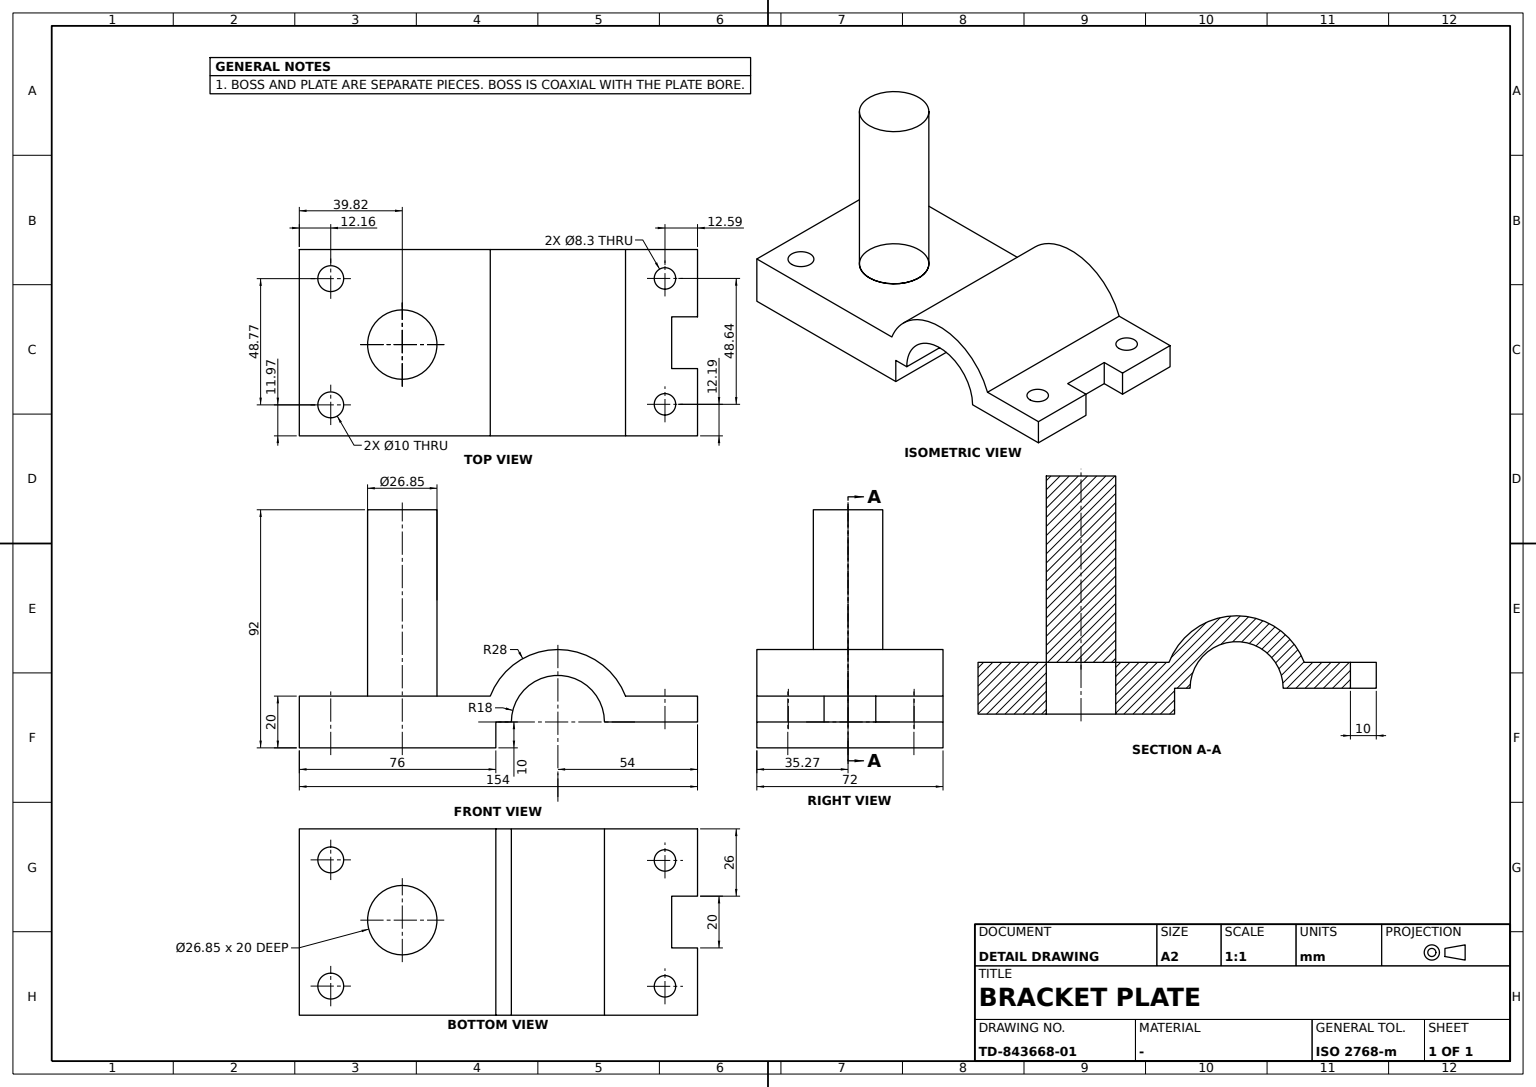
ISO-10303-21;
HEADER;
FILE_DESCRIPTION((''),'2;1');
FILE_NAME('','',(''),(''),'','','');
FILE_SCHEMA(('AUTOMOTIVE_DESIGN'));
ENDSEC;
DATA;
#1=APPLICATION_CONTEXT('');
#2=PRODUCT_CONTEXT('',#1,'mechanical');
#3=PRODUCT('','','',(#2));
#4=PRODUCT_DEFINITION_FORMATION('','',#3);
#5=PRODUCT_DEFINITION_CONTEXT('',#1,'design');
#6=PRODUCT_DEFINITION('','',#4,#5);
#7=PRODUCT_DEFINITION_SHAPE('','',#6);
#8=(LENGTH_UNIT()NAMED_UNIT(*)SI_UNIT(.MILLI.,.METRE.));
#9=(NAMED_UNIT(*)PLANE_ANGLE_UNIT()SI_UNIT($,.RADIAN.));
#10=(NAMED_UNIT(*)SI_UNIT($,.STERADIAN.)SOLID_ANGLE_UNIT());
#11=UNCERTAINTY_MEASURE_WITH_UNIT(LENGTH_MEASURE(0.005),#8,'distance_accuracy_value','');
#12=(GEOMETRIC_REPRESENTATION_CONTEXT(3)GLOBAL_UNCERTAINTY_ASSIGNED_CONTEXT((#11))GLOBAL_UNIT_ASSIGNED_CONTEXT((#8,#9,#10))REPRESENTATION_CONTEXT('',''));
#13=CARTESIAN_POINT('',(-21.846565,-37.180111,82.));
#14=VERTEX_POINT('',#13);
#15=CARTESIAN_POINT('',(-35.26936,-37.180111,82.));
#16=DIRECTION('',(0.,0.,1.));
#17=DIRECTION('',(1.,0.,0.));
#18=AXIS2_PLACEMENT_3D('',#15,#16,#17);
#19=CIRCLE('',#18,13.422795);
#20=EDGE_CURVE('',#14,#14,#19,.T.);
#21=ORIENTED_EDGE('',*,*,#20,.T.);
#22=EDGE_LOOP('',(#21));
#23=FACE_BOUND('',#22,.T.);
#24=CARTESIAN_POINT('',(0.,0.,82.));
#25=AXIS2_PLACEMENT_3D('',#24,#16,#17);
#26=PLANE('',#25);
#27=ADVANCED_FACE('',(#23),#26,.T.);
#28=CARTESIAN_POINT('',(-21.846565,-37.180111,10.));
#29=VERTEX_POINT('',#28);
#30=CARTESIAN_POINT('',(-35.26936,-37.180111,10.));
#31=AXIS2_PLACEMENT_3D('',#30,#16,#17);
#32=CIRCLE('',#31,13.422795);
#33=EDGE_CURVE('',#29,#29,#32,.T.);
#34=ORIENTED_EDGE('',*,*,#33,.F.);
#35=EDGE_LOOP('',(#34));
#36=FACE_BOUND('',#35,.T.);
#37=CARTESIAN_POINT('',(0.,49.153394,10.));
#38=DIRECTION('',(0.,1.,0.));
#39=AXIS2_PLACEMENT_3D('',#37,#16,#38);
#40=PLANE('',#39);
#41=ADVANCED_FACE('',(#36),#40,.F.);
#42=ORIENTED_EDGE('',*,*,#33,.T.);
#43=EDGE_LOOP('',(#42));
#44=FACE_BOUND('',#43,.T.);
#45=ORIENTED_EDGE('',*,*,#20,.F.);
#46=EDGE_LOOP('',(#45));
#47=FACE_BOUND('',#46,.T.);
#48=CARTESIAN_POINT('',(-35.26936,-37.180111,46.));
#49=AXIS2_PLACEMENT_3D('',#48,#16,#17);
#50=CYLINDRICAL_SURFACE('',#49,13.422795);
#51=ADVANCED_FACE('',(#44,#47),#50,.T.);
#52=CLOSED_SHELL('',(#27,#41,#51));
#53=MANIFOLD_SOLID_BREP('',#52);
#54=CARTESIAN_POINT('',(-48.692154,-37.180111,-10.));
#55=VERTEX_POINT('',#54);
#56=CARTESIAN_POINT('',(-35.26936,-37.180111,-10.));
#57=DIRECTION('',(0.,0.,-1.));
#58=DIRECTION('',(-1.,0.,0.));
#59=AXIS2_PLACEMENT_3D('',#56,#57,#58);
#60=CIRCLE('',#59,13.422795);
#61=EDGE_CURVE('',#55,#55,#60,.T.);
#62=ORIENTED_EDGE('',*,*,#61,.T.);
#63=EDGE_LOOP('',(#62));
#64=FACE_BOUND('',#63,.T.);
#65=VERTEX_POINT('',#28);
#66=EDGE_CURVE('',#65,#65,#32,.T.);
#67=ORIENTED_EDGE('',*,*,#66,.T.);
#68=EDGE_LOOP('',(#67));
#69=FACE_BOUND('',#68,.T.);
#70=ADVANCED_FACE('',(#64,#69),#50,.F.);
#71=CARTESIAN_POINT('',(0.,-1.,-10.));
#72=VERTEX_POINT('',#71);
#73=CARTESIAN_POINT('',(-72.,-1.,-10.));
#74=VERTEX_POINT('',#73);
#75=VECTOR('',#58,1000.);
#76=LINE('',#71,#75);
#77=EDGE_CURVE('',#72,#74,#76,.T.);
#78=ORIENTED_EDGE('',*,*,#77,.T.);
#79=CARTESIAN_POINT('',(-72.,-1.,0.));
#80=VERTEX_POINT('',#79);
#81=VECTOR('',#57,1000.);
#82=LINE('',#79,#81);
#83=EDGE_CURVE('',#80,#74,#82,.T.);
#84=ORIENTED_EDGE('',*,*,#83,.F.);
#85=CARTESIAN_POINT('',(0.,-1.,0.));
#86=VERTEX_POINT('',#85);
#87=LINE('',#85,#75);
#88=EDGE_CURVE('',#86,#80,#87,.T.);
#89=ORIENTED_EDGE('',*,*,#88,.F.);
#90=LINE('',#85,#81);
#91=EDGE_CURVE('',#86,#72,#90,.T.);
#92=ORIENTED_EDGE('',*,*,#91,.T.);
#93=EDGE_LOOP('',(#78,#84,#89,#92));
#94=FACE_BOUND('',#93,.T.);
#95=AXIS2_PLACEMENT_3D('',#85,#38,#57);
#96=PLANE('',#95);
#97=ADVANCED_FACE('',(#94),#96,.T.);
#98=CARTESIAN_POINT('',(0.,-77.,-10.));
#99=VERTEX_POINT('',#98);
#100=CARTESIAN_POINT('',(0.,-77.,10.));
#101=VERTEX_POINT('',#100);
#102=VECTOR('',#16,1000.);
#103=LINE('',#98,#102);
#104=EDGE_CURVE('',#99,#101,#103,.T.);
#105=ORIENTED_EDGE('',*,*,#104,.F.);
#106=DIRECTION('',(0.,-1.,0.));
#107=VECTOR('',#106,1000.);
#108=LINE('',#71,#107);
#109=EDGE_CURVE('',#72,#99,#108,.T.);
#110=ORIENTED_EDGE('',*,*,#109,.F.);
#111=ORIENTED_EDGE('',*,*,#91,.F.);
#112=CARTESIAN_POINT('',(0.,5.,0.));
#113=VERTEX_POINT('',#112);
#114=LINE('',#112,#107);
#115=EDGE_CURVE('',#113,#86,#114,.T.);
#116=ORIENTED_EDGE('',*,*,#115,.F.);
#117=CARTESIAN_POINT('',(0.,41.,0.));
#118=VERTEX_POINT('',#117);
#119=CARTESIAN_POINT('',(0.,23.,0.));
#120=AXIS2_PLACEMENT_3D('',#119,#17,#57);
#121=CIRCLE('',#120,18.);
#122=EDGE_CURVE('',#118,#113,#121,.T.);
#123=ORIENTED_EDGE('',*,*,#122,.F.);
#124=CARTESIAN_POINT('',(0.,77.,0.));
#125=VERTEX_POINT('',#124);
#126=EDGE_CURVE('',#125,#118,#114,.T.);
#127=ORIENTED_EDGE('',*,*,#126,.F.);
#128=CARTESIAN_POINT('',(0.,77.,10.));
#129=VERTEX_POINT('',#128);
#130=LINE('',#128,#81);
#131=EDGE_CURVE('',#129,#125,#130,.T.);
#132=ORIENTED_EDGE('',*,*,#131,.F.);
#133=VERTEX_POINT('',#37);
#134=VECTOR('',#38,1000.);
#135=LINE('',#37,#134);
#136=EDGE_CURVE('',#133,#129,#135,.T.);
#137=ORIENTED_EDGE('',*,*,#136,.F.);
#138=CARTESIAN_POINT('',(0.,-3.153394,10.));
#139=VERTEX_POINT('',#138);
#140=CIRCLE('',#120,28.);
#141=EDGE_CURVE('',#133,#139,#140,.T.);
#142=ORIENTED_EDGE('',*,*,#141,.T.);
#143=EDGE_CURVE('',#101,#139,#135,.T.);
#144=ORIENTED_EDGE('',*,*,#143,.F.);
#145=EDGE_LOOP('',(#105,#110,#111,#116,#123,#127,#132,#137,#142,#144));
#146=FACE_BOUND('',#145,.T.);
#147=CARTESIAN_POINT('',(0.,0.,0.));
#148=AXIS2_PLACEMENT_3D('',#147,#17,#38);
#149=PLANE('',#148);
#150=ADVANCED_FACE('',(#146),#149,.T.);
#151=CARTESIAN_POINT('',(-64.984131,64.410873,0.));
#152=VERTEX_POINT('',#151);
#153=CARTESIAN_POINT('',(-60.834221,64.410873,0.));
#154=AXIS2_PLACEMENT_3D('',#153,#57,#58);
#155=CIRCLE('',#154,4.14991);
#156=EDGE_CURVE('',#152,#152,#155,.T.);
#157=ORIENTED_EDGE('',*,*,#156,.T.);
#158=EDGE_LOOP('',(#157));
#159=FACE_BOUND('',#158,.T.);
#160=CARTESIAN_POINT('',(-56.684311,64.410873,10.));
#161=VERTEX_POINT('',#160);
#162=CARTESIAN_POINT('',(-60.834221,64.410873,10.));
#163=AXIS2_PLACEMENT_3D('',#162,#16,#17);
#164=CIRCLE('',#163,4.14991);
#165=EDGE_CURVE('',#161,#161,#164,.T.);
#166=ORIENTED_EDGE('',*,*,#165,.T.);
#167=EDGE_LOOP('',(#166));
#168=FACE_BOUND('',#167,.T.);
#169=CARTESIAN_POINT('',(-60.834221,64.410873,-26.));
#170=AXIS2_PLACEMENT_3D('',#169,#16,#17);
#171=CYLINDRICAL_SURFACE('',#170,4.14991);
#172=ADVANCED_FACE('',(#159,#168),#171,.F.);
#173=ORIENTED_EDGE('',*,*,#109,.T.);
#174=CARTESIAN_POINT('',(-72.,-77.,-10.));
#175=VERTEX_POINT('',#174);
#176=LINE('',#98,#75);
#177=EDGE_CURVE('',#99,#175,#176,.T.);
#178=ORIENTED_EDGE('',*,*,#177,.T.);
#179=LINE('',#73,#107);
#180=EDGE_CURVE('',#74,#175,#179,.T.);
#181=ORIENTED_EDGE('',*,*,#180,.F.);
#182=ORIENTED_EDGE('',*,*,#77,.F.);
#183=EDGE_LOOP('',(#173,#178,#181,#182));
#184=FACE_BOUND('',#183,.T.);
#185=ORIENTED_EDGE('',*,*,#61,.F.);
#186=EDGE_LOOP('',(#185));
#187=FACE_BOUND('',#186,.T.);
#188=CARTESIAN_POINT('',(-16.97486,-64.842331,-10.));
#189=VERTEX_POINT('',#188);
#190=CARTESIAN_POINT('',(-11.97486,-64.842331,-10.));
#191=AXIS2_PLACEMENT_3D('',#190,#57,#58);
#192=CIRCLE('',#191,5.);
#193=EDGE_CURVE('',#189,#189,#192,.T.);
#194=ORIENTED_EDGE('',*,*,#193,.F.);
#195=EDGE_LOOP('',(#194));
#196=FACE_BOUND('',#195,.T.);
#197=CARTESIAN_POINT('',(-65.747715,-64.842331,-10.));
#198=VERTEX_POINT('',#197);
#199=CARTESIAN_POINT('',(-60.747715,-64.842331,-10.));
#200=AXIS2_PLACEMENT_3D('',#199,#57,#58);
#201=CIRCLE('',#200,5.);
#202=EDGE_CURVE('',#198,#198,#201,.T.);
#203=ORIENTED_EDGE('',*,*,#202,.F.);
#204=EDGE_LOOP('',(#203));
#205=FACE_BOUND('',#204,.T.);
#206=AXIS2_PLACEMENT_3D('',#71,#57,#106);
#207=PLANE('',#206);
#208=ADVANCED_FACE('',(#184,#187,#196,#205),#207,.T.);
#209=ORIENTED_EDGE('',*,*,#122,.T.);
#210=CARTESIAN_POINT('',(-72.,5.,0.));
#211=VERTEX_POINT('',#210);
#212=VECTOR('',#17,1000.);
#213=LINE('',#112,#212);
#214=EDGE_CURVE('',#113,#211,#213,.F.);
#215=ORIENTED_EDGE('',*,*,#214,.T.);
#216=CARTESIAN_POINT('',(-72.,41.,0.));
#217=VERTEX_POINT('',#216);
#218=CARTESIAN_POINT('',(-72.,23.,0.));
#219=AXIS2_PLACEMENT_3D('',#218,#17,#57);
#220=CIRCLE('',#219,18.);
#221=EDGE_CURVE('',#217,#211,#220,.T.);
#222=ORIENTED_EDGE('',*,*,#221,.F.);
#223=LINE('',#117,#212);
#224=EDGE_CURVE('',#118,#217,#223,.F.);
#225=ORIENTED_EDGE('',*,*,#224,.F.);
#226=EDGE_LOOP('',(#209,#215,#222,#225));
#227=FACE_BOUND('',#226,.T.);
#228=CARTESIAN_POINT('',(-36.,23.,0.));
#229=AXIS2_PLACEMENT_3D('',#228,#17,#38);
#230=CYLINDRICAL_SURFACE('',#229,18.);
#231=ADVANCED_FACE('',(#227),#230,.F.);
#232=CARTESIAN_POINT('',(-55.747715,-64.842331,10.));
#233=VERTEX_POINT('',#232);
#234=CARTESIAN_POINT('',(-60.747715,-64.842331,10.));
#235=AXIS2_PLACEMENT_3D('',#234,#16,#17);
#236=CIRCLE('',#235,5.);
#237=EDGE_CURVE('',#233,#233,#236,.T.);
#238=ORIENTED_EDGE('',*,*,#237,.T.);
#239=EDGE_LOOP('',(#238));
#240=FACE_BOUND('',#239,.T.);
#241=ORIENTED_EDGE('',*,*,#202,.T.);
#242=EDGE_LOOP('',(#241));
#243=FACE_BOUND('',#242,.T.);
#244=CARTESIAN_POINT('',(-60.747715,-64.842331,-26.));
#245=AXIS2_PLACEMENT_3D('',#244,#16,#17);
#246=CYLINDRICAL_SURFACE('',#245,5.);
#247=ADVANCED_FACE('',(#240,#243),#246,.F.);
#248=CARTESIAN_POINT('',(-72.,-77.,10.));
#249=VERTEX_POINT('',#248);
#250=LINE('',#174,#102);
#251=EDGE_CURVE('',#175,#249,#250,.T.);
#252=ORIENTED_EDGE('',*,*,#251,.F.);
#253=ORIENTED_EDGE('',*,*,#177,.F.);
#254=ORIENTED_EDGE('',*,*,#104,.T.);
#255=LINE('',#100,#75);
#256=EDGE_CURVE('',#101,#249,#255,.T.);
#257=ORIENTED_EDGE('',*,*,#256,.T.);
#258=EDGE_LOOP('',(#252,#253,#254,#257));
#259=FACE_BOUND('',#258,.T.);
#260=AXIS2_PLACEMENT_3D('',#98,#106,#16);
#261=PLANE('',#260);
#262=ADVANCED_FACE('',(#259),#261,.T.);
#263=ORIENTED_EDGE('',*,*,#193,.T.);
#264=EDGE_LOOP('',(#263));
#265=FACE_BOUND('',#264,.T.);
#266=CARTESIAN_POINT('',(-6.97486,-64.842331,10.));
#267=VERTEX_POINT('',#266);
#268=CARTESIAN_POINT('',(-11.97486,-64.842331,10.));
#269=AXIS2_PLACEMENT_3D('',#268,#16,#17);
#270=CIRCLE('',#269,5.);
#271=EDGE_CURVE('',#267,#267,#270,.T.);
#272=ORIENTED_EDGE('',*,*,#271,.T.);
#273=EDGE_LOOP('',(#272));
#274=FACE_BOUND('',#273,.T.);
#275=CARTESIAN_POINT('',(-11.97486,-64.842331,-26.));
#276=AXIS2_PLACEMENT_3D('',#275,#16,#17);
#277=CYLINDRICAL_SURFACE('',#276,5.);
#278=ADVANCED_FACE('',(#265,#274),#277,.F.);
#279=ORIENTED_EDGE('',*,*,#271,.F.);
#280=EDGE_LOOP('',(#279));
#281=FACE_BOUND('',#280,.T.);
#282=ORIENTED_EDGE('',*,*,#256,.F.);
#283=ORIENTED_EDGE('',*,*,#143,.T.);
#284=CARTESIAN_POINT('',(-72.,-3.153394,10.));
#285=VERTEX_POINT('',#284);
#286=LINE('',#138,#212);
#287=EDGE_CURVE('',#139,#285,#286,.F.);
#288=ORIENTED_EDGE('',*,*,#287,.T.);
#289=CARTESIAN_POINT('',(-72.,49.153394,10.));
#290=LINE('',#289,#134);
#291=EDGE_CURVE('',#249,#285,#290,.T.);
#292=ORIENTED_EDGE('',*,*,#291,.F.);
#293=EDGE_LOOP('',(#282,#283,#288,#292));
#294=FACE_BOUND('',#293,.T.);
#295=ORIENTED_EDGE('',*,*,#66,.F.);
#296=EDGE_LOOP('',(#295));
#297=FACE_BOUND('',#296,.T.);
#298=ORIENTED_EDGE('',*,*,#237,.F.);
#299=EDGE_LOOP('',(#298));
#300=FACE_BOUND('',#299,.T.);
#301=ADVANCED_FACE('',(#281,#294,#297,#300),#40,.T.);
#302=ORIENTED_EDGE('',*,*,#287,.F.);
#303=ORIENTED_EDGE('',*,*,#141,.F.);
#304=VERTEX_POINT('',#289);
#305=LINE('',#37,#212);
#306=EDGE_CURVE('',#133,#304,#305,.F.);
#307=ORIENTED_EDGE('',*,*,#306,.T.);
#308=CIRCLE('',#219,28.);
#309=EDGE_CURVE('',#304,#285,#308,.T.);
#310=ORIENTED_EDGE('',*,*,#309,.T.);
#311=EDGE_LOOP('',(#302,#303,#307,#310));
#312=FACE_BOUND('',#311,.T.);
#313=CYLINDRICAL_SURFACE('',#229,28.);
#314=ADVANCED_FACE('',(#312),#313,.T.);
#315=CARTESIAN_POINT('',(-26.,77.,0.));
#316=VERTEX_POINT('',#315);
#317=LINE('',#124,#75);
#318=EDGE_CURVE('',#125,#316,#317,.T.);
#319=ORIENTED_EDGE('',*,*,#318,.T.);
#320=CARTESIAN_POINT('',(-26.,77.,10.));
#321=VERTEX_POINT('',#320);
#322=LINE('',#320,#81);
#323=EDGE_CURVE('',#321,#316,#322,.T.);
#324=ORIENTED_EDGE('',*,*,#323,.F.);
#325=LINE('',#128,#75);
#326=EDGE_CURVE('',#129,#321,#325,.T.);
#327=ORIENTED_EDGE('',*,*,#326,.F.);
#328=ORIENTED_EDGE('',*,*,#131,.T.);
#329=EDGE_LOOP('',(#319,#324,#327,#328));
#330=FACE_BOUND('',#329,.T.);
#331=AXIS2_PLACEMENT_3D('',#128,#38,#57);
#332=PLANE('',#331);
#333=ADVANCED_FACE('',(#330),#332,.T.);
#334=CARTESIAN_POINT('',(-26.,67.,10.));
#335=VERTEX_POINT('',#334);
#336=CARTESIAN_POINT('',(-26.,67.,0.));
#337=VERTEX_POINT('',#336);
#338=LINE('',#334,#81);
#339=EDGE_CURVE('',#335,#337,#338,.T.);
#340=ORIENTED_EDGE('',*,*,#339,.T.);
#341=CARTESIAN_POINT('',(-46.,67.,0.));
#342=VERTEX_POINT('',#341);
#343=CARTESIAN_POINT('',(0.,67.,0.));
#344=LINE('',#343,#75);
#345=EDGE_CURVE('',#337,#342,#344,.T.);
#346=ORIENTED_EDGE('',*,*,#345,.T.);
#347=CARTESIAN_POINT('',(-46.,67.,10.));
#348=VERTEX_POINT('',#347);
#349=LINE('',#347,#81);
#350=EDGE_CURVE('',#348,#342,#349,.T.);
#351=ORIENTED_EDGE('',*,*,#350,.F.);
#352=LINE('',#334,#75);
#353=EDGE_CURVE('',#335,#348,#352,.T.);
#354=ORIENTED_EDGE('',*,*,#353,.F.);
#355=EDGE_LOOP('',(#340,#346,#351,#354));
#356=FACE_BOUND('',#355,.T.);
#357=AXIS2_PLACEMENT_3D('',#334,#106,#58);
#358=PLANE('',#357);
#359=ADVANCED_FACE('',(#356),#358,.F.);
#360=ORIENTED_EDGE('',*,*,#339,.F.);
#361=LINE('',#320,#107);
#362=EDGE_CURVE('',#321,#335,#361,.T.);
#363=ORIENTED_EDGE('',*,*,#362,.F.);
#364=ORIENTED_EDGE('',*,*,#323,.T.);
#365=CARTESIAN_POINT('',(-26.,5.,0.));
#366=LINE('',#365,#107);
#367=EDGE_CURVE('',#316,#337,#366,.T.);
#368=ORIENTED_EDGE('',*,*,#367,.T.);
#369=EDGE_LOOP('',(#360,#363,#364,#368));
#370=FACE_BOUND('',#369,.T.);
#371=AXIS2_PLACEMENT_3D('',#320,#17,#106);
#372=PLANE('',#371);
#373=ADVANCED_FACE('',(#370),#372,.F.);
#374=ORIENTED_EDGE('',*,*,#214,.F.);
#375=ORIENTED_EDGE('',*,*,#115,.T.);
#376=ORIENTED_EDGE('',*,*,#88,.T.);
#377=LINE('',#210,#107);
#378=EDGE_CURVE('',#211,#80,#377,.T.);
#379=ORIENTED_EDGE('',*,*,#378,.F.);
#380=EDGE_LOOP('',(#374,#375,#376,#379));
#381=FACE_BOUND('',#380,.T.);
#382=AXIS2_PLACEMENT_3D('',#112,#57,#106);
#383=PLANE('',#382);
#384=ADVANCED_FACE('',(#381),#383,.T.);
#385=ORIENTED_EDGE('',*,*,#165,.F.);
#386=EDGE_LOOP('',(#385));
#387=FACE_BOUND('',#386,.T.);
#388=ORIENTED_EDGE('',*,*,#362,.T.);
#389=ORIENTED_EDGE('',*,*,#353,.T.);
#390=CARTESIAN_POINT('',(-46.,77.,10.));
#391=VERTEX_POINT('',#390);
#392=LINE('',#347,#134);
#393=EDGE_CURVE('',#348,#391,#392,.T.);
#394=ORIENTED_EDGE('',*,*,#393,.T.);
#395=CARTESIAN_POINT('',(-72.,77.,10.));
#396=VERTEX_POINT('',#395);
#397=EDGE_CURVE('',#391,#396,#325,.T.);
#398=ORIENTED_EDGE('',*,*,#397,.T.);
#399=EDGE_CURVE('',#304,#396,#290,.T.);
#400=ORIENTED_EDGE('',*,*,#399,.F.);
#401=ORIENTED_EDGE('',*,*,#306,.F.);
#402=ORIENTED_EDGE('',*,*,#136,.T.);
#403=ORIENTED_EDGE('',*,*,#326,.T.);
#404=EDGE_LOOP('',(#388,#389,#394,#398,#400,#401,#402,#403));
#405=FACE_BOUND('',#404,.T.);
#406=CARTESIAN_POINT('',(-8.042011,64.410873,10.));
#407=VERTEX_POINT('',#406);
#408=CARTESIAN_POINT('',(-12.191921,64.410873,10.));
#409=AXIS2_PLACEMENT_3D('',#408,#16,#17);
#410=CIRCLE('',#409,4.14991);
#411=EDGE_CURVE('',#407,#407,#410,.T.);
#412=ORIENTED_EDGE('',*,*,#411,.F.);
#413=EDGE_LOOP('',(#412));
#414=FACE_BOUND('',#413,.T.);
#415=ADVANCED_FACE('',(#387,#405,#414),#40,.T.);
#416=CARTESIAN_POINT('',(-16.341831,64.410873,0.));
#417=VERTEX_POINT('',#416);
#418=CARTESIAN_POINT('',(-12.191921,64.410873,0.));
#419=AXIS2_PLACEMENT_3D('',#418,#57,#58);
#420=CIRCLE('',#419,4.14991);
#421=EDGE_CURVE('',#417,#417,#420,.T.);
#422=ORIENTED_EDGE('',*,*,#421,.F.);
#423=EDGE_LOOP('',(#422));
#424=FACE_BOUND('',#423,.T.);
#425=ORIENTED_EDGE('',*,*,#367,.F.);
#426=ORIENTED_EDGE('',*,*,#318,.F.);
#427=ORIENTED_EDGE('',*,*,#126,.T.);
#428=ORIENTED_EDGE('',*,*,#224,.T.);
#429=CARTESIAN_POINT('',(-72.,77.,0.));
#430=VERTEX_POINT('',#429);
#431=EDGE_CURVE('',#430,#217,#377,.T.);
#432=ORIENTED_EDGE('',*,*,#431,.F.);
#433=CARTESIAN_POINT('',(-46.,77.,0.));
#434=VERTEX_POINT('',#433);
#435=EDGE_CURVE('',#434,#430,#317,.T.);
#436=ORIENTED_EDGE('',*,*,#435,.F.);
#437=LINE('',#341,#107);
#438=EDGE_CURVE('',#434,#342,#437,.T.);
#439=ORIENTED_EDGE('',*,*,#438,.T.);
#440=ORIENTED_EDGE('',*,*,#345,.F.);
#441=EDGE_LOOP('',(#425,#426,#427,#428,#432,#436,#439,#440));
#442=FACE_BOUND('',#441,.T.);
#443=ORIENTED_EDGE('',*,*,#156,.F.);
#444=EDGE_LOOP('',(#443));
#445=FACE_BOUND('',#444,.T.);
#446=ADVANCED_FACE('',(#424,#442,#445),#383,.T.);
#447=ORIENTED_EDGE('',*,*,#421,.T.);
#448=EDGE_LOOP('',(#447));
#449=FACE_BOUND('',#448,.T.);
#450=ORIENTED_EDGE('',*,*,#411,.T.);
#451=EDGE_LOOP('',(#450));
#452=FACE_BOUND('',#451,.T.);
#453=CARTESIAN_POINT('',(-12.191921,64.410873,-26.));
#454=AXIS2_PLACEMENT_3D('',#453,#16,#17);
#455=CYLINDRICAL_SURFACE('',#454,4.14991);
#456=ADVANCED_FACE('',(#449,#452),#455,.F.);
#457=ORIENTED_EDGE('',*,*,#435,.T.);
#458=LINE('',#395,#81);
#459=EDGE_CURVE('',#396,#430,#458,.T.);
#460=ORIENTED_EDGE('',*,*,#459,.F.);
#461=ORIENTED_EDGE('',*,*,#397,.F.);
#462=LINE('',#390,#81);
#463=EDGE_CURVE('',#391,#434,#462,.T.);
#464=ORIENTED_EDGE('',*,*,#463,.T.);
#465=EDGE_LOOP('',(#457,#460,#461,#464));
#466=FACE_BOUND('',#465,.T.);
#467=ADVANCED_FACE('',(#466),#332,.T.);
#468=ORIENTED_EDGE('',*,*,#83,.T.);
#469=ORIENTED_EDGE('',*,*,#180,.T.);
#470=ORIENTED_EDGE('',*,*,#251,.T.);
#471=ORIENTED_EDGE('',*,*,#291,.T.);
#472=ORIENTED_EDGE('',*,*,#309,.F.);
#473=ORIENTED_EDGE('',*,*,#399,.T.);
#474=ORIENTED_EDGE('',*,*,#459,.T.);
#475=ORIENTED_EDGE('',*,*,#431,.T.);
#476=ORIENTED_EDGE('',*,*,#221,.T.);
#477=ORIENTED_EDGE('',*,*,#378,.T.);
#478=EDGE_LOOP('',(#468,#469,#470,#471,#472,#473,#474,#475,#476,#477));
#479=FACE_BOUND('',#478,.T.);
#480=CARTESIAN_POINT('',(-72.,0.,0.));
#481=AXIS2_PLACEMENT_3D('',#480,#17,#38);
#482=PLANE('',#481);
#483=ADVANCED_FACE('',(#479),#482,.F.);
#484=ORIENTED_EDGE('',*,*,#393,.F.);
#485=ORIENTED_EDGE('',*,*,#350,.T.);
#486=ORIENTED_EDGE('',*,*,#438,.F.);
#487=ORIENTED_EDGE('',*,*,#463,.F.);
#488=EDGE_LOOP('',(#484,#485,#486,#487));
#489=FACE_BOUND('',#488,.T.);
#490=AXIS2_PLACEMENT_3D('',#347,#58,#38);
#491=PLANE('',#490);
#492=ADVANCED_FACE('',(#489),#491,.F.);
#493=CLOSED_SHELL('',(#70,#97,#150,#172,#208,#231,#247,#262,#278,#301,#314,#333,#359,#373,#384,#415,#446,#456,#467,#483,#492));
#494=MANIFOLD_SOLID_BREP('',#493);
#495=ADVANCED_BREP_SHAPE_REPRESENTATION('',(#53,#494),#12);
#496=SHAPE_DEFINITION_REPRESENTATION(#7,#495);
ENDSEC;
END-ISO-10303-21;
